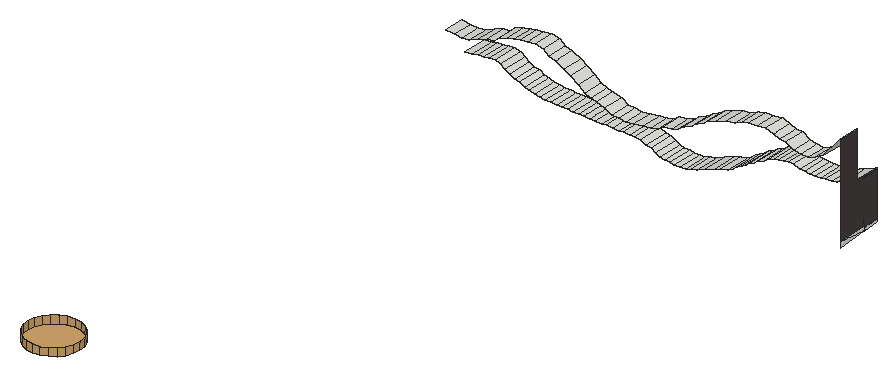
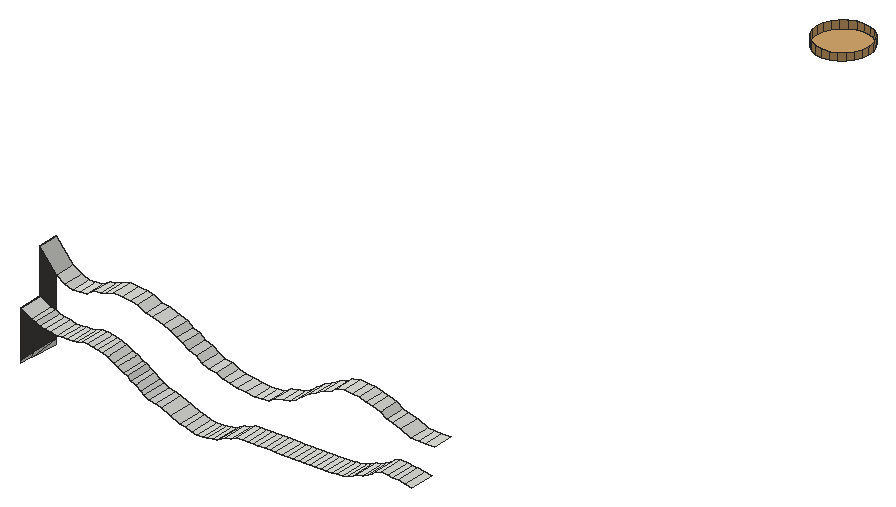
# SketchUp Ruby script. Lengths in inches.
U = 1.inch
M = Sketchup.active_model
def pt(a) = Geom::Point3d.new(a.map { |v| v * U })
def face(e, loops, mat)
  f = e.add_face(loops[0].map { |a| pt(a) })
  loops[1..].each { |l| e.add_face(l.map { |a| pt(a) }).erase! }
  f.material = f.back_material = mat if mat
  f
end
# faces: each face lists its corners as indices into pts; further lists are holes
def faces(e, pts, list, mat = nil) = list.each { |f| face(e, (f[0].is_a?(Array) ? f : [f]).map { |l| l.map { |i| pts[i] } }, mat) }
# xy, xz, yz: faces in a plane at the given z, y or x. An outline is a flat list of corners, or four numbers for a rectangle; further outlines are holes
def ring(l) = l.size == 4 ? [[l[0], l[1]], [l[2], l[1]], [l[2], l[3]], [l[0], l[3]]] : l.each_slice(2).to_a
def flat(e, list, mat, &to3) = list.each { |f| face(e, (f[0].is_a?(Array) ? f : [f]).map { |l| ring(l).map { |u, v| to3.(u, v) } }, mat) }
def xy(e, z, list, mat = nil) = flat(e, list, mat) { |x, y| [x, y, z] }
def xz(e, y, list, mat = nil) = flat(e, list, mat) { |x, z| [x, y, z] }
def yz(e, x, list, mat = nil) = flat(e, list, mat) { |y, z| [x, y, z] }
def lines(e, pts, list) = list.each { |a, b| e.add_line(pt(pts[a]), pt(pts[b])) }
# prism: a flat outline (further loops are holes) pulled along v
def prism(e, loops, v, mat = nil)
  f = face(e, loops, mat); d = Geom::Vector3d.new(v.map { |x| x * U })
  f.pushpull(f.normal.samedirection?(d) ? d.length : -d.length)
end
def box(e, o, s, mat = nil) = prism(e, [[o, [o[0] + s[0], o[1], o[2]], [o[0] + s[0], o[1] + s[1], o[2]], [o[0], o[1] + s[1], o[2]]]], [0, 0, s[2]], mat)
def at(x, y, z, deg = 0) = Geom::Transformation.translation(pt([x, y, z])) * Geom::Transformation.rotation(ORIGIN, Z_AXIS, deg.degrees)
def axes(o, x, y, z) = Geom::Transformation.new([*x, 0, *y, 0, *z, 0, *pt(o).to_a, 1])
def part(name) = M.definitions.add(name)
# library, detail: a bought-in or finely detailed component or shape, given as its bounding box
def library(name, o, s) = part(name).tap { |d| box(d.entities, o, s) }
def detail(e, o, s) = box(e.add_group.entities, o, s)
def put(e, d, t, mat = nil) = e.add_instance(d, t).tap { |i| i.material = mat if mat }
def group(e, t, mat = nil) = e.add_group.tap { |g| g.transformation = t; g.material = mat if mat }.entities
root = M.entities
M.materials.add("[Field Square Tile]").color = [211, 167, 108]
M.materials.add("[Granite Tile]1").color = [68, 65, 63]
xy(root,250.6875,[[377.043,2328.207,376.331,2328.3,375.668,2328.575,375.098,2329.012,374.661,2329.582,374.386,2330.245,374.293,2330.957,374.386,2331.668,374.661,2332.332,375.098,2332.901,375.668,2333.338,376.331,2333.613,377.043,2333.707,377.754,2333.613,378.418,2333.338,378.987,2332.901,379.424,2332.332,379.699,2331.668,379.793,2330.957,379.699,2330.245,379.424,2329.582,378.987,2329.012,378.418,2328.575,377.754,2328.3]],"[Field Square Tile]")
yz(root,406.845,[[2396.678,240.932,2396.678,241.519,2399.776,241.17],[2399.81,241.167,2399.776,241.17,2399.809,241.173],[2399.776,241.17,2396.678,241.519,2399.769,241.519,2399.809,241.173],[2399.809,241.173,2399.769,241.519,2401.365,241.519,2401.365,241.293]])
yz(root,406.845,[[2396.678,241.519,2396.678,251.165,2398.803,251.165,2398.803,246.426,2401.365,246.426,2401.365,241.519]],"[Granite Tile]1")
p = [[387.267,2398.803,241.17],[387.267,2401.365,241.17],[387.737,2401.365,241.121],[387.737,2398.803,241.121],[388.343,2401.365,241.09],[388.343,2398.803,241.09],
  [388.91,2401.365,241.138],[388.91,2398.803,241.138],[389.55,2401.365,241.346],[389.55,2398.803,241.346],[386.269,2398.803,241.332],[386.269,2401.365,241.332],
  [386.737,2401.365,241.243],[386.737,2398.803,241.243],[385.85,2398.803,241.566],[385.85,2401.365,241.566],[390.141,2401.365,241.456],[390.141,2398.803,241.456],
  [391.076,2401.365,241.847],[391.076,2398.803,241.847],[385.344,2398.803,241.837],[385.344,2401.365,241.837],[384.771,2398.803,241.967],[384.771,2401.365,241.967],
  [392.081,2401.365,242.229],[392.081,2398.803,242.229],[384.19,2398.803,242.199],[384.19,2401.365,242.199],[383.564,2398.803,242.277],[383.564,2401.365,242.277],
  [392.642,2401.365,242.424],[392.642,2398.803,242.424],[377.717,2398.803,242.35],[377.717,2401.365,242.35],[378.299,2401.365,242.342],[378.299,2398.803,242.342],
  [378.881,2401.365,242.334],[378.881,2398.803,242.334],[379.463,2401.365,242.326],[379.463,2398.803,242.326],[380.183,2401.365,242.317],[380.183,2398.803,242.317],
  [380.653,2401.365,242.312],[380.653,2398.803,242.312],[381.294,2401.365,242.304],[381.294,2398.803,242.304],[381.958,2401.365,242.296],[381.958,2398.803,242.296],
  [382.41,2401.365,242.291],[382.41,2398.803,242.291],[383.048,2401.365,242.283],[383.048,2398.803,242.283],[374.235,2398.803,242.466],[374.235,2401.365,242.466],
  [374.811,2401.365,242.428],[374.811,2398.803,242.428],[375.39,2401.365,242.403],[375.39,2398.803,242.403],[375.97,2401.365,242.385],[375.97,2398.803,242.385],
  [376.552,2401.365,242.371],[376.552,2398.803,242.371],[377.134,2401.365,242.36],[377.134,2398.803,242.36],[393.36,2401.365,242.605],[393.36,2398.803,242.605],
  [373.107,2398.803,242.599],[373.107,2401.365,242.599],[373.667,2401.365,242.518],[373.667,2398.803,242.518],[372.554,2398.803,242.75],[372.554,2401.365,242.75],
  [393.873,2401.365,242.907],[393.873,2398.803,242.907],[372.066,2398.803,242.921],[372.066,2401.365,242.921],[371.575,2398.803,243.216],[371.575,2401.365,243.216],
  [394.245,2401.365,243.144],[394.245,2398.803,243.144],[394.794,2401.365,243.516],[394.794,2398.803,243.516],[371.027,2398.803,243.332],[371.027,2401.365,243.332],
  [370.482,2398.803,243.589],[370.482,2401.365,243.589],[395.268,2401.365,243.711],[395.268,2398.803,243.711],[370.001,2398.803,243.88],[370.001,2401.365,243.88],
  [395.599,2401.365,244.02],[395.599,2398.803,244.02],[369.624,2398.803,244.194],[369.624,2401.365,244.194],[365.836,2398.803,243.992],[365.836,2401.365,243.992],
  [366.539,2401.365,244.076],[366.539,2398.803,244.076],[396.043,2401.365,244.206],[396.043,2398.803,244.206],[367.238,2401.365,244.207],[367.238,2398.803,244.207],
  [367.823,2401.365,244.266],[367.823,2398.803,244.266],[369.027,2398.803,244.387],[369.027,2401.365,244.387],[396.632,2401.365,244.569],[396.632,2398.803,244.569],
  [368.364,2401.365,244.296],[368.364,2398.803,244.296],[397.102,2401.365,244.757],[397.102,2398.803,244.757],[397.719,2401.365,245.125],[397.719,2398.803,245.125],
  [382.915,2396.678,245.064],[382.915,2398.803,245.064],[383.625,2398.803,244.949],[383.625,2396.678,244.949],[384.339,2398.803,244.867],[384.339,2396.678,244.867],
  [385.245,2398.803,245.007],[385.245,2396.678,245.007],[386.189,2398.803,245.121],[386.189,2396.678,245.121],[382.202,2396.678,245.459],[382.202,2398.803,245.459],
  [386.954,2398.803,245.254],[386.954,2396.678,245.254],[398.223,2401.365,245.32],[398.223,2398.803,245.32],[401.924,2398.803,245.272],[401.924,2401.365,245.272],
  [402.482,2401.365,245.235],[402.482,2398.803,245.235],[403.036,2401.365,245.216],[403.036,2398.803,245.216],[403.601,2401.365,245.34],[403.601,2398.803,245.34],
  [387.706,2398.803,245.41],[387.706,2396.678,245.41],[398.705,2401.365,245.411],[398.705,2398.803,245.411],[400.271,2398.803,245.552],[400.271,2401.365,245.552],
  [400.879,2401.365,245.346],[400.879,2398.803,245.346],[401.373,2401.365,245.309],[401.373,2398.803,245.309],[404.233,2401.365,245.423],[404.233,2398.803,245.423],
  [388.34,2398.803,245.775],[388.34,2396.678,245.775],[399.253,2401.365,245.481],[399.253,2398.803,245.481],[404.811,2401.365,245.516],[404.811,2398.803,245.516],
  [381.327,2396.678,245.671],[381.327,2398.803,245.671],[399.735,2401.365,245.59],[399.735,2398.803,245.59],[405.191,2401.365,245.763],[405.191,2398.803,245.763],
  [380.652,2396.678,245.834],[380.652,2398.803,245.834],[380.064,2396.678,246.129],[380.064,2398.803,246.129],[389.136,2398.803,245.88],[389.136,2396.678,245.88],
  [405.66,2401.365,245.896],[405.66,2398.803,245.896],[389.849,2398.803,246.16],[389.849,2396.678,246.16],[406.845,2401.365,246.426],[406.845,2398.803,246.426],
  [379.433,2396.678,246.633],[379.433,2398.803,246.633],[390.446,2398.803,246.573],[390.446,2396.678,246.573],[378.619,2396.678,247.185],[378.619,2398.803,247.185],
  [391.236,2398.803,246.902],[391.236,2396.678,246.902],[366.442,2396.678,246.79],[366.442,2398.803,246.79],[367.221,2398.803,246.747],[367.221,2396.678,246.747],
  [367.968,2398.803,246.831],[367.968,2396.678,246.831],[365.488,2396.678,246.838],[365.488,2398.803,246.838],[369.01,2398.803,247.251],[369.01,2396.678,247.251],
  [391.838,2398.803,247.347],[391.838,2396.678,247.347],[377.907,2396.678,247.553],[377.907,2398.803,247.553],[369.884,2398.803,247.546],[369.884,2396.678,247.546],
  [392.512,2398.803,247.615],[392.512,2396.678,247.615],[370.546,2398.803,247.657],[370.546,2396.678,247.657],[377.016,2396.678,248.059],[377.016,2398.803,248.059],
  [393.099,2398.803,248.057],[393.099,2396.678,248.057],[371.179,2398.803,248.162],[371.179,2396.678,248.162],[376.325,2396.678,248.257],[376.325,2398.803,248.257],
  [393.864,2398.803,248.322],[393.864,2396.678,248.322],[371.973,2398.803,248.408],[371.973,2396.678,248.408],[402.661,2396.678,248.295],[402.661,2398.803,248.295],
  [403.37,2398.803,248.218],[403.37,2396.678,248.218],[404.187,2398.803,248.558],[404.187,2396.678,248.558],[375.794,2396.678,248.687],[375.794,2398.803,248.687],
  [394.975,2398.803,248.655],[394.975,2396.678,248.655],[401.95,2396.678,248.42],[401.95,2398.803,248.42],[372.672,2398.803,248.521],[372.672,2396.678,248.521],
  [401.153,2396.678,248.895],[401.153,2398.803,248.895],[373.366,2398.803,248.723],[373.366,2396.678,248.723],[405.122,2398.803,249.022],[405.122,2396.678,249.022],
  [374.065,2398.803,248.801],[374.065,2396.678,248.801],[374.962,2396.678,248.851],[374.962,2398.803,248.851],[395.748,2398.803,248.795],[395.748,2396.678,248.795],
  [396.611,2398.803,249.194],[396.611,2396.678,249.194],[400.449,2396.678,248.962],[400.449,2398.803,248.962],[399.81,2396.678,249.206],[399.81,2398.803,249.206],
  [406.845,2398.803,251.165],[406.845,2396.678,251.165],[397.284,2398.803,249.323],[397.284,2396.678,249.323],[399.065,2396.678,249.478],[399.065,2398.803,249.478],
  [398.207,2398.803,249.406],[398.207,2396.678,249.406],[377.043,2328.207,251.5],[376.331,2328.3,251.5],[376.331,2328.3,250.6875],[377.043,2328.207,250.6875],
  [377.754,2328.3,251.5],[377.754,2328.3,250.6875],[375.668,2328.575,251.5],[375.668,2328.575,250.6875],[378.418,2328.575,251.5],[378.418,2328.575,250.6875],
  [375.098,2329.012,251.5],[375.098,2329.012,250.6875],[378.987,2329.012,251.5],[378.987,2329.012,250.6875],[374.661,2329.582,251.5],[374.661,2329.582,250.6875],
  [379.424,2329.582,251.5],[379.424,2329.582,250.6875],[374.386,2330.245,251.5],[374.386,2330.245,250.6875],[379.699,2330.245,251.5],[379.699,2330.245,250.6875],
  [374.293,2330.957,251.5],[374.293,2330.957,250.6875],[379.793,2330.957,251.5],[379.793,2330.957,250.6875],[374.386,2331.668,251.5],[374.386,2331.668,250.6875],
  [379.699,2331.668,251.5],[379.699,2331.668,250.6875],[374.661,2332.332,251.5],[374.661,2332.332,250.6875],[379.424,2332.332,251.5],[379.424,2332.332,250.6875],
  [375.098,2332.901,251.5],[375.098,2332.901,250.6875],[378.987,2332.901,251.5],[378.987,2332.901,250.6875],[375.668,2333.338,251.5],[375.668,2333.338,250.6875],
  [378.418,2333.338,251.5],[378.418,2333.338,250.6875],[376.331,2333.613,251.5],[376.331,2333.613,250.6875],[377.754,2333.613,251.5],[377.754,2333.613,250.6875],
  [377.043,2333.707,251.5],[377.043,2333.707,250.6875],[406.845,2400.588,246.171],[406.845,2399.573,246.265],[406.845,2401.365,246.273],[406.845,2399.769,241.519],
  [406.845,2399.667,242.384]]
faces(root,p,[[0,1,2,3],[3,2,4,5],[5,4,6,7],[7,6,8,9],[10,11,12,13],[13,12,1,0],[14,15,11,10],[9,8,16,17],
  [17,16,18,19],[20,21,15,14],[22,23,21,20],[19,18,24,25],[26,27,23,22],[28,29,27,26],[25,24,30,31],[32,33,34,35],
  [35,34,36,37],[37,36,38,39],[39,38,40,41],[41,40,42,43],[43,42,44,45],[45,44,46,47],[47,46,48,49],[49,48,50,51],
  [51,50,29,28],[52,53,54,55],[55,54,56,57],[57,56,58,59],[59,58,60,61],[61,60,62,63],[63,62,33,32],[31,30,64,65],
  [66,67,68,69],[69,68,53,52],[70,71,67,66],[65,64,72,73],[74,75,71,70],[76,77,75,74],[73,72,78,79],[79,78,80,81],
  [82,83,77,76],[84,85,83,82],[81,80,86,87],[88,89,85,84],[87,86,90,91],[92,93,89,88],[94,95,96,97],[91,90,98,99],
  [97,96,100,101],[101,100,102,103],[104,105,93,92],[99,98,106,107],[103,102,108,109],[109,108,105,104],[107,106,110,111],[111,110,112,113],
  [114,115,116,117],[117,116,118,119],[119,118,120,121],[121,120,122,123],[124,125,115,114],[123,122,126,127],[113,112,128,129],[130,131,132,133],
  [133,132,134,135],[135,134,136,137],[127,126,138,139],[129,128,140,141],[142,143,144,145],[145,144,146,147],[147,146,131,130],[137,136,148,149],
  [139,138,150,151],[141,140,152,153],[149,148,154,155],[156,157,125,124],[153,152,158,159],[155,154,160,161],[159,158,143,142],[162,163,157,156],
  [164,165,163,162],[151,150,166,167],[161,160,168,169],[167,166,170,171],[169,168,172,173],[174,175,165,164],[171,170,176,177],[178,179,175,174],
  [177,176,180,181],[182,183,184,185],[185,184,186,187],[188,189,183,182],[187,186,190,191],[181,180,192,193],[194,195,179,178],[191,190,196,197],
  [193,192,198,199],[197,196,200,201],[202,203,195,194],[199,198,204,205],[201,200,206,207],[208,209,203,202],[205,204,210,211],[207,206,212,213],
  [214,215,216,217],[217,216,218,219],[220,221,209,208],[211,210,222,223],[224,225,215,214],[213,212,226,227],[228,229,225,224],[227,226,230,231],
  [219,218,232,233],[231,230,234,235],[236,237,221,220],[223,222,238,239],[235,234,237,236],[239,238,240,241],[242,243,229,228],[244,245,243,242],
  [233,232,246,247],[241,240,248,249],[250,251,245,244],[249,248,252,253],[253,252,251,250]])
faces(root,p,[[254,255,256,257],[258,254,257,259],[255,260,261,256],[262,258,259,263],[260,264,265,261],[266,262,263,267],[264,268,269,265],[270,266,267,271],
  [268,272,273,269],[274,270,271,275],[272,276,277,273],[278,274,275,279],[276,280,281,277],[282,278,279,283],[280,284,285,281],[286,282,283,287],
  [284,288,289,285],[290,286,287,291],[288,292,293,289],[294,290,291,295],[292,296,297,293],[298,294,295,299],[296,300,301,297],[300,298,299,301]],"[Field Square Tile]")
lines(root,p,[[302,303],[304,302],[305,306]])
